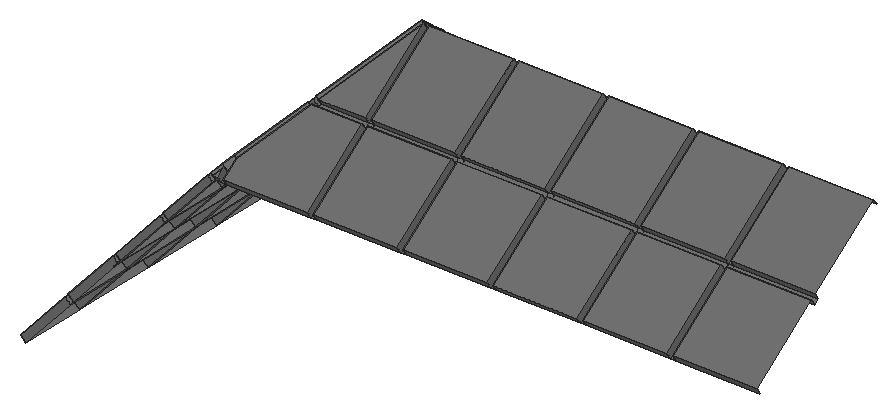
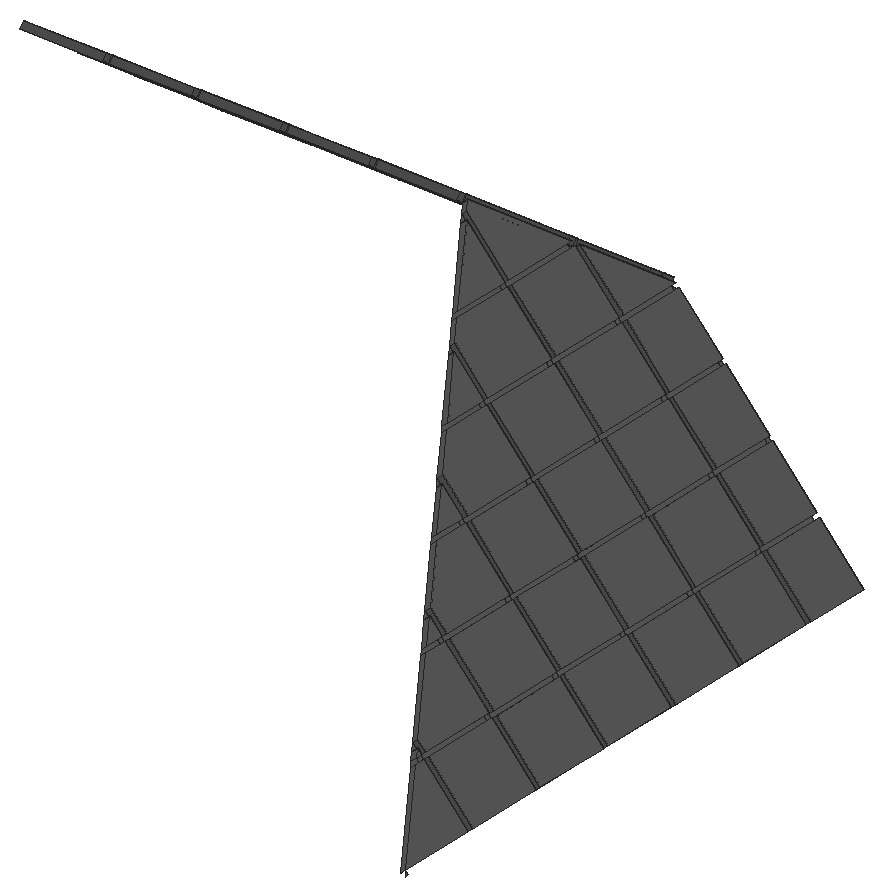
# SketchUp Ruby script. Lengths in inches.
U = 1.inch
M = Sketchup.active_model
def pt(a) = Geom::Point3d.new(a.map { |v| v * U })
def face(e, loops, mat)
  f = e.add_face(loops[0].map { |a| pt(a) })
  loops[1..].each { |l| e.add_face(l.map { |a| pt(a) }).erase! }
  f.material = f.back_material = mat if mat
  f
end
# faces: each face lists its corners as indices into pts; further lists are holes
def faces(e, pts, list, mat = nil) = list.each { |f| face(e, (f[0].is_a?(Array) ? f : [f]).map { |l| l.map { |i| pts[i] } }, mat) }
# xy, xz, yz: faces in a plane at the given z, y or x. An outline is a flat list of corners, or four numbers for a rectangle; further outlines are holes
def ring(l) = l.size == 4 ? [[l[0], l[1]], [l[2], l[1]], [l[2], l[3]], [l[0], l[3]]] : l.each_slice(2).to_a
def flat(e, list, mat, &to3) = list.each { |f| face(e, (f[0].is_a?(Array) ? f : [f]).map { |l| ring(l).map { |u, v| to3.(u, v) } }, mat) }
def xy(e, z, list, mat = nil) = flat(e, list, mat) { |x, y| [x, y, z] }
def xz(e, y, list, mat = nil) = flat(e, list, mat) { |x, z| [x, y, z] }
def yz(e, x, list, mat = nil) = flat(e, list, mat) { |y, z| [x, y, z] }
def lines(e, pts, list) = list.each { |a, b| e.add_line(pt(pts[a]), pt(pts[b])) }
# prism: a flat outline (further loops are holes) pulled along v
def prism(e, loops, v, mat = nil)
  f = face(e, loops, mat); d = Geom::Vector3d.new(v.map { |x| x * U })
  f.pushpull(f.normal.samedirection?(d) ? d.length : -d.length)
end
def box(e, o, s, mat = nil) = prism(e, [[o, [o[0] + s[0], o[1], o[2]], [o[0] + s[0], o[1] + s[1], o[2]], [o[0], o[1] + s[1], o[2]]]], [0, 0, s[2]], mat)
def at(x, y, z, deg = 0) = Geom::Transformation.translation(pt([x, y, z])) * Geom::Transformation.rotation(ORIGIN, Z_AXIS, deg.degrees)
def axes(o, x, y, z) = Geom::Transformation.new([*x, 0, *y, 0, *z, 0, *pt(o).to_a, 1])
def part(name) = M.definitions.add(name)
# library, detail: a bought-in or finely detailed component or shape, given as its bounding box
def library(name, o, s) = part(name).tap { |d| box(d.entities, o, s) }
def detail(e, o, s) = box(e.add_group.entities, o, s)
def put(e, d, t, mat = nil) = e.add_instance(d, t).tap { |i| i.material = mat if mat }
def group(e, t, mat = nil) = e.add_group.tap { |g| g.transformation = t; g.material = mat if mat }.entities
root = M.entities
M.materials.add("[Color M05]").color = [114, 114, 114]
xz(root,415.43,[[371.99,444.64,383.89,457.92,382.4,459.26,370.5,445.97],[384.68,458.81,396.57,472.1,395.08,473.43,383.1875,460.14],[397.37,472.98,409.26,486.27,407.77,487.6,395.88,474.32],[410.06,487.15,421.95,500.4375,420.46,501.77,408.57,488.49]],"[Color M05]")
xz(root,433.3,[[371.99,444.64,370.5,445.97,382.4,459.26,383.89,457.92],[384.68,458.81,383.1875,460.14,395.08,473.43,396.57,472.1],[397.37,472.98,395.88,474.32,407.77,487.6,409.26,486.27],[410.06,487.15,408.57,488.49,420.46,501.77,421.95,500.4375],[422.75,501.32,421.26,502.66,432.96,515.73,434.45,514.4]],"[Color M05]")
xz(root,434.8,[[371.99,444.64,383.89,457.92,382.4,459.26,370.5,445.97],[384.68,458.81,396.57,472.1,395.08,473.43,383.1875,460.14],[397.37,472.98,409.26,486.27,407.77,487.6,395.88,474.32],[410.06,487.15,421.95,500.4375,420.46,501.77,408.57,488.49],[422.75,501.32,434.64,514.61,433.15,515.94,421.26,502.66]],"[Color M05]")
xz(root,456.21,[[371.99,444.64,370.5,445.97,382.4,459.26,383.89,457.92],[384.68,458.81,383.1875,460.14,395.08,473.43,396.57,472.1],[397.37,472.98,395.88,474.32,407.77,487.6,409.26,486.27],[410.06,487.15,408.57,488.49,420.46,501.77,421.95,500.4375],[422.75,501.32,421.26,502.66,433.15,515.94,434.64,514.61],
  [435.43,515.5,433.94,516.83,445.29,529.51,446.78,528.17]],"[Color M05]")
xz(root,457.71,[[371.99,444.64,383.89,457.92,382.4,459.26,370.5,445.97],[384.68,458.81,396.57,472.1,395.08,473.43,383.1875,460.14],[397.37,472.98,409.26,486.27,407.77,487.6,395.88,474.32],[410.06,487.15,421.95,500.4375,420.46,501.77,408.57,488.49],[422.75,501.32,434.64,514.61,433.15,515.94,421.26,502.66],
  [435.43,515.5,445.8,527.07,444.3125,528.41,433.94,516.83]],"[Color M05]")
xz(root,479.13,[[371.99,444.64,370.5,445.97,382.4,459.26,383.89,457.92],[384.68,458.81,383.1875,460.14,395.08,473.43,396.57,472.1],[397.37,472.98,395.88,474.32,407.77,487.6,409.26,486.27],[410.06,487.15,408.57,488.49,420.46,501.77,421.95,500.4375],[422.75,501.32,421.26,502.66,430.28,512.74,431.77,511.41]],"[Color M05]")
xz(root,480.63,[[371.99,444.64,383.89,457.92,382.4,459.26,370.5,445.97],[384.68,458.81,396.57,472.1,395.08,473.43,383.1875,460.14],[397.37,472.98,409.26,486.27,407.77,487.6,395.88,474.32],[410.06,487.15,421.95,500.4375,420.46,501.77,408.57,488.49],[422.75,501.32,430.79,510.31,429.3,511.64,421.26,502.66]],"[Color M05]")
xz(root,502.04,[[371.99,444.64,370.5,445.97,382.4,459.26,383.89,457.92],[384.68,458.81,383.1875,460.14,395.08,473.43,396.57,472.1],[397.37,472.98,395.88,474.32,407.77,487.6,409.26,486.27],[410.06,487.15,408.57,488.49,415.27,495.98,416.76,494.64]],"[Color M05]")
xz(root,503.54,[[371.99,444.64,383.89,457.92,382.4,459.26,370.5,445.97],[384.68,458.81,396.57,472.1,395.08,473.43,383.1875,460.14],[397.37,472.98,409.26,486.27,407.77,487.6,395.88,474.32],[410.06,487.15,415.78,493.55,414.29,494.88,408.57,488.49]],"[Color M05]")
xz(root,524.95,[[371.99,444.64,370.5,445.97,382.4,459.26,383.89,457.92],[384.68,458.81,383.1875,460.14,395.08,473.43,396.57,472.1],[397.37,472.98,395.88,474.32,400.26,479.21,401.75,477.88]],"[Color M05]")
xz(root,526.45,[[371.99,444.64,383.89,457.92,382.4,459.26,370.5,445.97],[384.68,458.81,396.57,472.1,395.08,473.43,383.1875,460.14],[397.37,472.98,400.77,476.78,399.28,478.12,395.88,474.32]],"[Color M05]")
xz(root,547.87,[[371.99,444.64,370.5,445.97,382.4,459.26,383.89,457.92],[384.68,458.81,383.1875,460.14,385.25,462.45,386.74,461.11]],"[Color M05]")
xz(root,549.37,[[371.99,444.64,383.89,457.92,382.4,459.26,370.5,445.97],[384.68,458.81,385.76,460.02,384.27,461.35,383.1875,460.14]],"[Color M05]")
yz(root,424.12,[[415.43,501.32,417.53,502.86,416.35,504.48,414.25,502.9375]],"[Color M05]")
yz(root,425.62,[[415.43,501.32,414.25,502.9375,418.64,506.15,419.82,504.54]],"[Color M05]")
yz(root,448.12,[[415.43,501.32,433.59,514.61,432.41,516.22,414.25,502.9375],[434.8,515.5,454.17,529.67,452.99,531.28,433.62,517.11]],"[Color M05]")
yz(root,449.62,[[415.43,501.32,414.25,502.9375,432.41,516.22,433.59,514.61],[434.8,515.5,433.62,517.11,452.99,531.28,454.17,529.67]],"[Color M05]")
yz(root,472.12,[[415.43,501.32,433.59,514.61,432.41,516.22,414.25,502.9375],[434.8,515.5,454.17,529.67,452.99,531.28,433.62,517.11]],"[Color M05]")
yz(root,473.62,[[415.43,501.32,414.25,502.9375,432.41,516.22,433.59,514.61],[434.8,515.5,433.62,517.11,452.99,531.28,454.17,529.67]],"[Color M05]")
yz(root,496.12,[[415.43,501.32,433.59,514.61,432.41,516.22,414.25,502.9375],[434.8,515.5,454.17,529.67,452.99,531.28,433.62,517.11]],"[Color M05]")
yz(root,497.62,[[415.43,501.32,414.25,502.9375,432.41,516.22,433.59,514.61],[434.8,515.5,433.62,517.11,452.99,531.28,454.17,529.67]],"[Color M05]")
yz(root,520.12,[[415.43,501.32,433.59,514.61,432.41,516.22,414.25,502.9375],[434.8,515.5,454.17,529.67,452.99,531.28,433.62,517.11]],"[Color M05]")
yz(root,521.62,[[415.43,501.32,414.25,502.9375,432.41,516.22,433.59,514.61],[434.8,515.5,433.62,517.11,452.99,531.28,454.17,529.67]],"[Color M05]")
yz(root,544.12,[[415.43,501.32,433.59,514.61,432.41,516.22,414.25,502.9375],[434.8,515.5,454.17,529.67,452.99,531.28,433.62,517.11]],"[Color M05]")
yz(root,545.62,[[415.43,501.32,414.25,502.9375,432.41,516.22,433.59,514.61],[434.8,515.5,433.62,517.11,452.99,531.28,454.17,529.67]],"[Color M05]")
p = [[371.99,433.3,444.64],[371.99,415.43,444.64],[370.5,415.43,445.97],[370.5,433.3,445.97],[371.99,434.8,444.64],[383.89,433.3,457.92],
  [383.89,434.8,457.92],[371.99,456.21,444.64],[370.5,434.8,445.97],[370.5,456.21,445.97],[371.99,457.71,444.64],[383.89,456.21,457.92],
  [383.89,457.71,457.92],[371.99,479.13,444.64],[370.5,457.71,445.97],[370.5,479.13,445.97],[371.99,480.63,444.64],[383.89,479.13,457.92],
  [383.89,480.63,457.92],[371.99,502.04,444.64],[370.5,480.63,445.97],[370.5,502.04,445.97],[371.99,503.54,444.64],[383.89,502.04,457.92],
  [383.89,503.54,457.92],[371.99,524.95,444.64],[370.5,503.54,445.97],[370.5,524.95,445.97],[371.99,526.45,444.64],[383.89,524.95,457.92],
  [383.89,526.45,457.92],[371.99,547.87,444.64],[370.5,526.45,445.97],[370.5,547.87,445.97],[371.99,549.37,444.64],[383.89,547.87,457.92],
  [383.89,549.37,457.92],[371.99,570.39,444.64],[370.5,549.37,445.97],[370.5,570.39,445.97],[383.89,552.23,457.92],[382.4,552.23,459.26],
  [369.71,571.6,445.09],[369.71,570.78,445.09],[370.24,570.78,445.68],[382.4,415.43,459.26],[382.4,433.3,459.26],[382.4,434.8,459.26],
  [382.4,456.21,459.26],[382.4,457.71,459.26],[382.4,479.13,459.26],[382.4,480.63,459.26],[382.4,502.04,459.26],[382.4,503.54,459.26],
  [382.4,524.95,459.26],[382.4,526.45,459.26],[382.4,547.87,459.26],[382.4,549.37,459.26],[383.89,415.43,457.92],[384.68,415.43,458.81],
  [384.68,433.3,458.81],[384.68,434.8,458.81],[384.68,456.21,458.81],[384.68,457.71,458.81],[384.68,479.13,458.81],[384.68,480.63,458.81],
  [384.68,502.04,458.81],[384.68,503.54,458.81],[384.68,524.95,458.81],[384.68,526.45,458.81],[384.68,547.87,458.81],[384.68,549.37,458.81],
  [384.68,551.02,458.81],[383.1875,415.43,460.14],[383.1875,433.3,460.14],[396.57,433.3,472.1],[396.57,434.8,472.1],[383.1875,434.8,460.14],
  [383.1875,456.21,460.14],[396.57,456.21,472.1],[396.57,457.71,472.1],[383.1875,457.71,460.14],[383.1875,479.13,460.14],[396.57,479.13,472.1],
  [396.57,480.63,472.1],[383.1875,480.63,460.14],[383.1875,502.04,460.14],[396.57,502.04,472.1],[396.57,503.54,472.1],[383.1875,503.54,460.14],
  [383.1875,524.95,460.14],[396.57,524.95,472.1],[396.57,526.45,472.1],[383.1875,526.45,460.14],[383.1875,547.87,460.14],[386.74,547.87,461.11],
  [385.76,549.37,460.02],[383.1875,549.37,460.14],[383.1875,551.02,460.14],[384.27,549.37,461.35],[395.08,415.43,473.43],[395.08,433.3,473.43],
  [395.08,434.8,473.43],[395.08,456.21,473.43],[395.08,457.71,473.43],[395.08,479.13,473.43],[395.08,480.63,473.43],[395.08,502.04,473.43],
  [395.08,503.54,473.43],[395.08,524.95,473.43],[395.08,526.45,473.43],[395.08,532.86,473.43],[385.25,547.87,462.45],[396.57,532.86,472.1],
  [396.57,415.43,472.1],[396.57,414.22,472.1],[397.37,414.22,472.98],[397.37,415.43,472.98],[397.37,433.3,472.98],[397.37,434.8,472.98],
  [397.37,456.21,472.98],[397.37,457.71,472.98],[397.37,479.13,472.98],[397.37,480.63,472.98],[397.37,502.04,472.98],[397.37,503.54,472.98],
  [397.37,524.95,472.98],[397.37,526.45,472.98],[397.37,531.65,472.98],[409.26,414.22,486.27],[409.26,415.43,486.27],[395.88,415.43,474.32],
  [395.88,433.3,474.32],[409.26,433.3,486.27],[409.26,434.8,486.27],[395.88,434.8,474.32],[395.88,456.21,474.32],[409.26,456.21,486.27],
  [409.26,457.71,486.27],[395.88,457.71,474.32],[395.88,479.13,474.32],[409.26,479.13,486.27],[409.26,480.63,486.27],[395.88,480.63,474.32],
  [395.88,502.04,474.32],[409.26,502.04,486.27],[409.26,503.54,486.27],[395.88,503.54,474.32],[395.88,524.95,474.32],[401.75,524.95,477.88],
  [400.77,526.45,476.78],[395.88,526.45,474.32],[395.88,531.65,474.32],[399.28,526.45,478.12],[407.77,415.43,487.6],[407.77,433.3,487.6],
  [407.77,434.8,487.6],[407.77,456.21,487.6],[407.77,457.71,487.6],[407.77,479.13,487.6],[407.77,480.63,487.6],[407.77,502.04,487.6],
  [407.77,503.54,487.6],[407.77,513.49,487.6],[400.26,524.95,479.21],[409.26,513.49,486.27],[410.06,414.22,487.15],[410.06,415.43,487.15],
  [410.06,433.3,487.15],[410.06,434.8,487.15],[410.06,456.21,487.15],[410.06,457.71,487.15],[410.06,479.13,487.15],[410.06,480.63,487.15],
  [410.06,502.04,487.15],[410.06,503.54,487.15],[410.06,512.28,487.15],[421.95,414.22,500.4375],[421.95,415.43,500.4375],[408.57,415.43,488.49],
  [408.57,433.3,488.49],[421.95,433.3,500.4375],[421.95,434.8,500.4375],[408.57,434.8,488.49],[408.57,456.21,488.49],[421.95,456.21,500.4375],
  [421.95,457.71,500.4375],[408.57,457.71,488.49],[408.57,479.13,488.49],[421.95,479.13,500.4375],[421.95,480.63,500.4375],[408.57,480.63,488.49],
  [408.57,502.04,488.49],[416.76,502.04,494.64],[415.78,503.54,493.55],[408.57,503.54,488.49],[408.57,512.28,488.49],[414.29,503.54,494.88],
  [420.46,415.43,501.77],[420.46,433.3,501.77],[420.46,434.8,501.77],[420.46,456.21,501.77],[420.46,457.71,501.77],[420.46,479.13,501.77],
  [420.46,480.63,501.77],[420.46,494.12,501.77],[415.27,502.04,495.98],[421.95,494.12,500.4375],[422.75,415.43,501.32],[422.75,433.3,501.32],
  [422.75,434.8,501.32],[422.75,456.21,501.32],[422.75,457.71,501.32],[422.75,479.13,501.32],[422.75,480.63,501.32],[422.75,492.91,501.32],
  [424.12,415.43,501.32],[424.12,414.25,502.9375],[422.75,414.25,502.9375],[424.12,417.53,502.86],[424.12,416.35,504.48],[425.62,415.43,501.32],
  [448.12,415.43,501.32],[448.12,414.25,502.9375],[425.62,414.25,502.9375],[449.62,415.43,501.32],[472.12,415.43,501.32],[472.12,414.25,502.9375],
  [449.62,414.25,502.9375],[473.62,415.43,501.32],[496.12,415.43,501.32],[496.12,414.25,502.9375],[473.62,414.25,502.9375],[497.62,415.43,501.32],
  [520.12,415.43,501.32],[520.12,414.25,502.9375],[497.62,414.25,502.9375],[521.62,415.43,501.32],[544.12,415.43,501.32],[544.12,414.25,502.9375],
  [521.62,414.25,502.9375],[545.62,415.43,501.32],[568.12,415.43,501.32],[568.12,414.25,502.9375],[545.62,414.25,502.9375],[422.63,417.53,504.2],
  [421.26,415.43,502.66],[421.26,433.3,502.66],[425.62,419.82,504.54],[449.62,433.59,514.61],[448.12,433.59,514.61],[473.62,433.59,514.61],
  [472.12,433.59,514.61],[497.62,433.59,514.61],[496.12,433.59,514.61],[521.62,433.59,514.61],[520.12,433.59,514.61],[545.62,433.59,514.61],
  [544.12,433.59,514.61],[434.45,433.3,514.4],[434.64,433.59,514.61],[434.64,434.8,514.61],[421.26,434.8,502.66],[421.26,456.21,502.66],
  [434.64,456.21,514.61],[434.64,457.71,514.61],[421.26,457.71,502.66],[421.26,479.13,502.66],[431.77,479.13,511.41],[430.79,480.63,510.31],
  [421.26,480.63,502.66],[421.26,492.91,502.66],[429.3,480.63,511.64],[424.13,419.82,505.87],[432.96,433.3,515.73],[433.15,434.8,515.94],
  [433.15,456.21,515.94],[433.15,457.71,515.94],[433.15,474.75,515.94],[430.28,479.13,512.74],[448.12,432.41,516.22],[434.64,432.41,516.22],
  [434.45,432.12,516.01],[425.62,418.64,506.15],[472.12,432.41,516.22],[449.62,432.41,516.22],[496.12,432.41,516.22],[473.62,432.41,516.22],
  [520.12,432.41,516.22],[497.62,432.41,516.22],[544.12,432.41,516.22],[521.62,432.41,516.22],[568.12,432.41,516.22],[545.62,432.41,516.22],
  [434.64,474.75,514.61],[568.12,433.59,514.61],[448.12,434.8,515.5],[435.43,434.8,515.5],[449.62,434.8,515.5],[472.12,434.8,515.5],
  [473.62,434.8,515.5],[496.12,434.8,515.5],[497.62,434.8,515.5],[520.12,434.8,515.5],[521.62,434.8,515.5],[544.12,434.8,515.5],
  [545.62,434.8,515.5],[568.12,434.8,515.5],[435.43,456.21,515.5],[435.43,457.71,515.5],[435.43,473.54,515.5],[448.12,433.62,517.11],
  [435.43,433.62,517.11],[448.12,454.17,529.67],[448.12,452.99,531.28],[472.12,433.62,517.11],[449.62,433.62,517.11],[496.12,433.62,517.11],
  [473.62,433.62,517.11],[520.12,433.62,517.11],[497.62,433.62,517.11],[544.12,433.62,517.11],[521.62,433.62,517.11],[568.12,433.62,517.11],
  [545.62,433.62,517.11],[446.63,454.17,531],[433.94,434.8,516.83],[433.94,456.21,516.83],[449.62,454.17,529.67],[473.62,454.17,529.67],
  [472.12,454.17,529.67],[497.62,454.17,529.67],[496.12,454.17,529.67],[521.62,454.17,529.67],[520.12,454.17,529.67],[545.62,454.17,529.67],
  [544.12,454.17,529.67],[446.78,456.21,528.17],[445.8,457.71,527.07],[433.94,457.71,516.83],[433.94,473.54,516.83],[444.3125,457.71,528.41],
  [445.29,456.21,529.51],[472.12,452.99,531.28],[449.62,452.99,531.28],[496.12,452.99,531.28],[473.62,452.99,531.28],[520.12,452.99,531.28],
  [497.62,452.99,531.28],[544.12,452.99,531.28],[521.62,452.99,531.28],[568.12,452.99,531.28],[545.62,452.99,531.28],[568.12,454.17,529.67]]
faces(root,p,[[0,1,2,3],[4,0,5,6],[7,4,8,9],[10,7,11,12],[13,10,14,15],[16,13,17,18],[19,16,20,21],[22,19,23,24],
  [25,22,26,27],[28,25,29,30],[31,28,32,33],[34,31,35,36],[37,34,38,39],[40,37,39,41],[42,43,44],[3,2,45,46],
  [47,48,9,8],[15,14,49,50],[21,20,51,52],[27,26,53,54],[33,32,55,56],[39,38,57,41],[58,5,46,45],[5,58,59,60],
  [6,5,60,61],[6,11,48,47],[61,62,11,6],[12,11,62,63],[12,17,50,49],[17,12,63,64],[18,17,64,65],[18,23,52,51],
  [23,18,65,66],[24,23,66,67],[24,29,54,53],[29,24,67,68],[30,29,68,69],[30,35,56,55],[35,30,69,70],[36,35,70,71],
  [36,40,41,57],[40,36,71,72],[60,59,73,74],[61,60,75,76],[62,61,77,78],[63,62,79,80],[64,63,81,82],[65,64,83,84],
  [66,65,85,86],[67,66,87,88],[68,67,89,90],[69,68,91,92],[70,69,93,94],[71,70,95,96],[72,71,97,98],[96,72,98,99],
  [74,73,100,101],[102,103,78,77],[82,81,104,105],[86,85,106,107],[90,89,108,109],[94,93,110,111,112],[98,97,99],[113,95,112,111],
  [114,115,116,117],[114,75,101,100],[75,114,117,118],[76,75,118,119],[76,79,103,102],[119,120,79,76],[80,79,120,121],[80,83,105,104],
  [83,80,121,122],[84,83,122,123],[84,87,107,106],[87,84,123,124],[88,87,124,125],[88,91,109,108],[91,88,125,126],[92,91,126,127],
  [92,113,111,110],[113,92,127,128],[117,116,129,130],[118,117,131,132],[119,118,133,134],[120,119,135,136],[121,120,137,138],[122,121,139,140],
  [123,122,141,142],[124,123,143,144],[125,124,145,146],[126,125,147,148],[127,126,149,150],[128,127,151,152],[150,128,152,153],[132,131,154,155],
  [156,157,136,135],[140,139,158,159],[144,143,160,161],[148,147,162,163,164],[152,151,153],[165,149,164,163],[130,129,166,167],[130,133,155,154],
  [133,130,167,168],[134,133,168,169],[134,137,157,156],[169,170,137,134],[138,137,170,171],[138,141,159,158],[141,138,171,172],[142,141,172,173],
  [142,145,161,160],[145,142,173,174],[146,145,174,175],[146,165,163,162],[165,146,175,176],[167,166,177,178],[168,167,179,180],[169,168,181,182],
  [170,169,183,184],[171,170,185,186],[172,171,187,188],[173,172,189,190],[174,173,191,192],[175,174,193,194],[176,175,195,196],[194,176,196,197],
  [180,179,198,199],[200,201,184,183],[188,187,202,203],[192,191,204,205,206],[196,195,197],[207,193,206,205],[177,208,178],[178,181,199,198],
  [181,178,208,209],[182,181,209,210],[182,185,201,200],[210,211,185,182],[186,185,211,212],[186,189,203,202],[189,186,212,213],[190,189,213,214],
  [190,207,205,204],[207,190,214,215],[208,216,217,218],[219,208,218,220],[221,222,223,224],[225,226,227,228],[229,230,231,232],[233,234,235,236],
  [237,238,239,240],[241,242,243,244],[208,219,245,246],[209,208,246,247],[216,221,248,219],[222,225,249,250],[226,229,251,252],[230,233,253,254],
  [234,237,255,256],[238,241,257,258],[210,209,259,260,261],[211,210,262,263],[212,211,264,265],[213,212,266,267],[214,213,268,269],[215,214,270,271],
  [269,215,271,272],[273,274,247,246,245],[275,276,263,262],[267,266,277,278,279],[271,270,272],[218,217,220],[224,223,280,281,282,283],[228,227,284,285],
  [232,231,286,287],[236,235,288,289],[240,239,290,291],[244,243,292,293],[219,248,273,245],[259,248,283,282],[248,259,274,273],[294,268,279,278],
  [260,259,282,281],[250,260,281,280],[252,249,285,284],[254,251,287,286],[256,253,289,288],[258,255,291,290],[295,257,293,292],[260,250,296,297],
  [260,297,261],[250,249,298,296],[249,252,299,298],[252,251,300,299],[251,254,301,300],[254,253,302,301],[253,256,303,302],[256,255,304,303],
  [255,258,305,304],[258,257,306,305],[257,295,307,306],[261,264,276,275],[297,308,264,261],[265,264,308,309],[265,294,278,277],[294,265,309,310],
  [297,296,311,312],[313,297,312,314],[298,299,315,316],[300,301,317,318],[302,303,319,320],[304,305,321,322],[306,307,323,324],[297,313,325,326],
  [308,297,326,327],[296,298,328,313],[299,300,329,330],[301,302,331,332],[303,304,333,334],[305,306,335,336],[309,308,337,338],[310,309,339,340],
  [338,310,340,341],[325,342,327,326],[340,339,341],[312,311,314],[316,315,343,344],[318,317,345,346],[320,319,347,348],[322,321,349,350],
  [324,323,351,352],[313,337,342,325],[330,328,344,343],[332,329,346,345],[334,331,348,347],[336,333,350,349],[353,335,352,351]],"[Color M05]")
